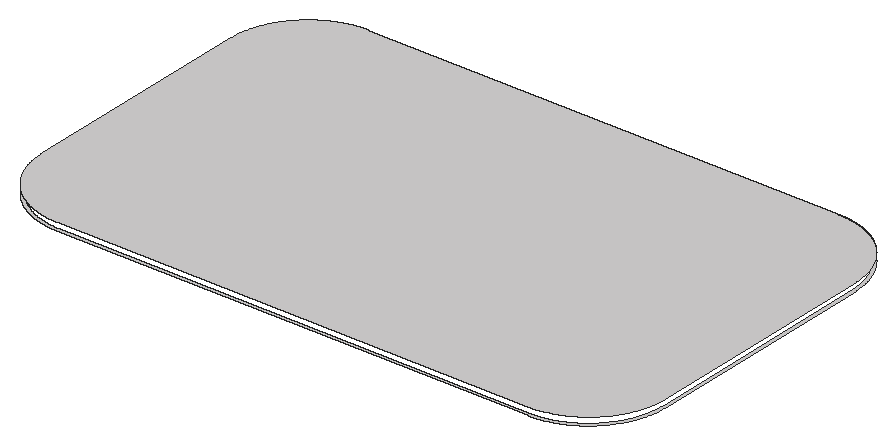
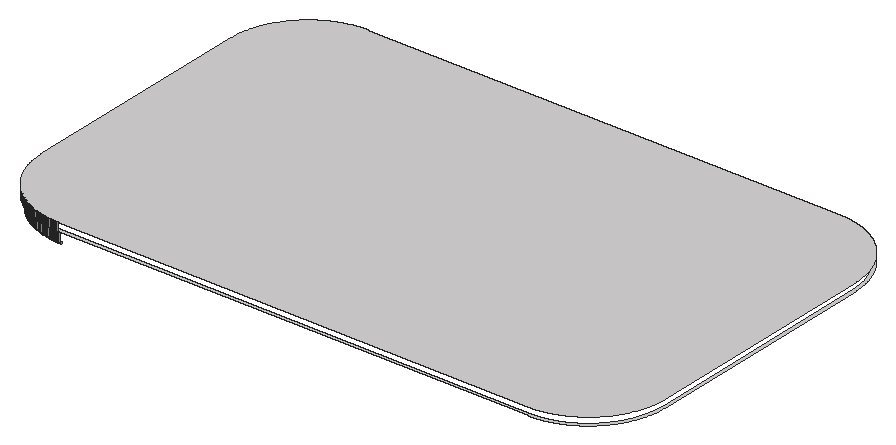
# SketchUp Ruby script. Lengths in inches.
U = 1.inch
M = Sketchup.active_model
def pt(a) = Geom::Point3d.new(a.map { |v| v * U })
def face(e, loops, mat)
  f = e.add_face(loops[0].map { |a| pt(a) })
  loops[1..].each { |l| e.add_face(l.map { |a| pt(a) }).erase! }
  f.material = f.back_material = mat if mat
  f
end
# faces: each face lists its corners as indices into pts; further lists are holes
def faces(e, pts, list, mat = nil) = list.each { |f| face(e, (f[0].is_a?(Array) ? f : [f]).map { |l| l.map { |i| pts[i] } }, mat) }
# xy, xz, yz: faces in a plane at the given z, y or x. An outline is a flat list of corners, or four numbers for a rectangle; further outlines are holes
def ring(l) = l.size == 4 ? [[l[0], l[1]], [l[2], l[1]], [l[2], l[3]], [l[0], l[3]]] : l.each_slice(2).to_a
def flat(e, list, mat, &to3) = list.each { |f| face(e, (f[0].is_a?(Array) ? f : [f]).map { |l| ring(l).map { |u, v| to3.(u, v) } }, mat) }
def xy(e, z, list, mat = nil) = flat(e, list, mat) { |x, y| [x, y, z] }
def xz(e, y, list, mat = nil) = flat(e, list, mat) { |x, z| [x, y, z] }
def yz(e, x, list, mat = nil) = flat(e, list, mat) { |y, z| [x, y, z] }
def lines(e, pts, list) = list.each { |a, b| e.add_line(pt(pts[a]), pt(pts[b])) }
# prism: a flat outline (further loops are holes) pulled along v
def prism(e, loops, v, mat = nil)
  f = face(e, loops, mat); d = Geom::Vector3d.new(v.map { |x| x * U })
  f.pushpull(f.normal.samedirection?(d) ? d.length : -d.length)
end
def box(e, o, s, mat = nil) = prism(e, [[o, [o[0] + s[0], o[1], o[2]], [o[0] + s[0], o[1] + s[1], o[2]], [o[0], o[1] + s[1], o[2]]]], [0, 0, s[2]], mat)
def at(x, y, z, deg = 0) = Geom::Transformation.translation(pt([x, y, z])) * Geom::Transformation.rotation(ORIGIN, Z_AXIS, deg.degrees)
def axes(o, x, y, z) = Geom::Transformation.new([*x, 0, *y, 0, *z, 0, *pt(o).to_a, 1])
def part(name) = M.definitions.add(name)
# library, detail: a bought-in or finely detailed component or shape, given as its bounding box
def library(name, o, s) = part(name).tap { |d| box(d.entities, o, s) }
def detail(e, o, s) = box(e.add_group.entities, o, s)
def put(e, d, t, mat = nil) = e.add_instance(d, t).tap { |i| i.material = mat if mat }
def group(e, t, mat = nil) = e.add_group.tap { |g| g.transformation = t; g.material = mat if mat }.entities
root = M.entities
M.materials.add("[Quartz Light Brown]").color = [215, 212, 212]
xy(root,493,[[[224.48,281.2,223.97,281.21,223.45,281.23,222.93,281.26,222.42,281.29,221.9,281.32,221.39,281.37,220.87,281.42,220.36,281.47,219.84,281.54,219.33,281.61,218.82,281.6875,218.3125,281.77,217.8,281.86,217.29,281.96,216.79,282.0625,216.28,282.17,215.78,282.29,214.28,282.68,213.78,282.83,213.29,282.98,212.79,283.13,211.81,283.47,211.33,283.64,210.84,283.82,210.36,284.01,209.88,284.21,209.41,284.41,208.93,284.62,208.46,284.83,207.99,285.05,207.53,285.27,207.07,285.51,206.61,285.74,206.15,285.99,205.25,286.49,204.8,286.75,203.92,287.29,203.49,287.57,203.05,287.86,202.2,288.44,201.78,288.74,201.37,289.05,200.95,289.36,200.55,289.68,200.14,290,199.74,290.33,199.35,290.66,198.96,291,198.57,291.35,198.1875,291.7,197.81,292.05,197.4375,292.41,197.07,292.77,196.35,293.51,195.99,293.89,195.65,294.27,195.3,294.66,194.96,295.05,194.63,295.44,194.3,295.84,193.98,296.25,193.66,296.65,193.35,297.07,193.04,297.48,192.74,297.9,192.16,298.76,191.87,299.1875,191.59,299.625,191.05,300.5,190.79,300.95,190.29,301.85,190.04,302.31,189.81,302.77,189.57,303.23,189.35,303.7,189.13,304.16,188.91,304.63,188.51,305.59,188.3125,306.0625,188.125,306.55,187.94,307.03,187.77,307.52,187.6,308,187.43,308.49,187.28,308.99,187.125,309.48,186.98,309.98,186.59,311.48,186.47,311.98,186.36,312.49,186.26,312.99,186.16,313.5,186.07,314.01,185.91,315.03,185.84,315.55,185.77,316.06,185.72,316.57,185.67,317.09,185.62,317.6,185.58,318.12,185.55,318.63,185.51,319.67,185.5,320.18,185.5,441.22,185.51,441.73,185.55,442.77,185.58,443.28,185.62,443.8,185.67,444.32,185.77,445.34,185.84,445.86,185.91,446.37,186.07,447.39,186.16,447.9,186.26,448.41,186.36,448.91,186.47,449.42,186.59,449.92,186.98,451.42,187.125,451.92,187.28,452.41,187.43,452.91,187.77,453.89,187.94,454.37,188.125,454.86,188.3125,455.34,188.51,455.82,188.71,456.29,188.91,456.77,189.35,457.71,189.57,458.17,189.81,458.63,190.04,459.09,190.29,459.55,190.79,460.45,191.05,460.9,191.59,461.78,191.87,462.21,192.16,462.65,192.45,463.07,192.74,463.5,193.04,463.92,193.35,464.33,193.66,464.75,193.98,465.16,194.3,465.56,194.63,465.96,194.96,466.35,195.3,466.75,195.65,467.13,195.99,467.51,196.35,467.89,197.07,468.63,197.4375,468.99,197.81,469.35,198.1875,469.71,198.57,470.06,199.35,470.74,199.74,471.07,200.14,471.4,200.55,471.72,200.95,472.04,201.37,472.35,201.78,472.66,202.2,472.96,203.05,473.54,203.49,473.83,203.92,474.11,204.8,474.65,205.25,474.91,206.15,475.41,206.61,475.66,207.07,475.9,207.53,476.13,207.99,476.35,208.93,476.79,209.41,476.99,209.88,477.19,210.36,477.39,210.84,477.58,211.33,477.76,211.81,477.94,212.3,478.1,212.79,478.27,213.29,478.42,213.78,478.57,214.28,478.72,214.78,478.86,215.28,478.99,216.28,479.23,216.79,479.34,217.29,479.44,217.8,479.54,218.3125,479.63,218.82,479.71,219.33,479.79,219.84,479.86,220.36,479.93,220.87,479.98,221.39,480.04,221.9,480.08,222.42,480.12,222.93,480.15,223.45,480.17,223.97,480.1875,224.48,480.2,464.52,480.2,465.03,480.1875,465.55,480.17,466.07,480.15,466.58,480.12,467.1,480.08,467.61,480.04,468.13,479.98,468.64,479.93,469.16,479.86,469.67,479.79,470.18,479.71,470.6875,479.63,471.2,479.54,471.71,479.44,472.21,479.34,472.72,479.23,473.72,478.99,474.22,478.86,474.72,478.72,475.22,478.57,475.71,478.42,476.21,478.27,476.7,478.1,477.19,477.94,477.67,477.76,478.16,477.58,478.64,477.39,479.12,477.19,479.59,476.99,480.07,476.79,481.01,476.35,481.47,476.13,481.93,475.9,482.39,475.66,482.85,475.41,483.75,474.91,484.2,474.65,485.08,474.11,485.51,473.83,485.95,473.54,486.8,472.96,487.22,472.66,487.63,472.35,488.05,472.04,488.45,471.72,488.86,471.4,489.26,471.07,489.65,470.74,490.43,470.06,490.8125,469.71,491.19,469.35,491.5625,468.99,491.93,468.63,492.65,467.89,493.01,467.51,493.35,467.13,493.7,466.75,494.04,466.35,494.37,465.96,494.7,465.56,495.02,465.16,495.34,464.75,495.65,464.33,495.96,463.92,496.26,463.5,496.55,463.07,496.84,462.65,497.13,462.21,497.41,461.78,497.95,460.9,498.21,460.45,498.71,459.55,498.96,459.09,499.19,458.63,499.43,458.17,499.65,457.71,500.09,456.77,500.29,456.29,500.49,455.82,500.6875,455.34,500.875,454.86,501.06,454.37,501.23,453.89,501.57,452.91,501.72,452.41,501.875,451.92,502.02,451.42,502.41,449.92,502.53,449.42,502.64,448.91,502.74,448.41,502.84,447.9,502.93,447.39,503.09,446.37,503.16,445.86,503.23,445.34,503.33,444.32,503.38,443.8,503.42,443.28,503.45,442.77,503.49,441.73,503.5,441.22,503.5,320.18,503.49,319.67,503.45,318.63,503.42,318.12,503.38,317.6,503.33,317.09,503.28,316.57,503.23,316.06,503.16,315.55,503.09,315.03,502.93,314.01,502.84,313.5,502.74,312.99,502.64,312.49,502.53,311.98,502.41,311.48,502.02,309.98,501.875,309.48,501.72,308.99,501.57,308.49,501.4,308,501.23,307.52,501.06,307.03,500.875,306.55,500.6875,306.0625,500.49,305.59,500.09,304.63,499.87,304.16,499.65,303.7,499.43,303.23,499.19,302.77,498.96,302.31,498.71,301.85,498.21,300.95,497.95,300.5,497.41,299.625,497.13,299.1875,496.84,298.76,496.26,297.9,495.96,297.48,495.65,297.07,495.34,296.65,495.02,296.25,494.7,295.84,494.37,295.44,494.04,295.05,493.7,294.66,493.35,294.27,493.01,293.89,492.65,293.51,491.93,292.77,491.5625,292.41,491.19,292.05,490.8125,291.7,490.43,291.35,490.04,291,489.65,290.66,489.26,290.33,488.86,290,488.45,289.68,488.05,289.36,487.63,289.05,487.22,288.74,486.8,288.44,485.95,287.86,485.51,287.57,485.08,287.29,484.2,286.75,483.75,286.49,482.85,285.99,482.39,285.74,481.93,285.51,481.47,285.27,481.01,285.05,480.54,284.83,480.07,284.62,479.59,284.41,479.12,284.21,478.64,284.01,478.16,283.82,477.67,283.64,477.19,283.47,476.21,283.13,475.71,282.98,475.22,282.83,474.72,282.68,473.22,282.29,472.72,282.17,472.21,282.0625,471.71,281.96,471.2,281.86,470.6875,281.77,470.18,281.6875,469.67,281.61,469.16,281.54,468.64,281.47,468.13,281.42,467.61,281.37,467.1,281.32,466.58,281.29,466.07,281.26,465.55,281.23,465.03,281.21,464.52,281.2],[224.5,282.7,464.5,282.7,464.99,282.71,465.99,282.75,466.49,282.78,466.98,282.82,467.48,282.86,467.97,282.91,468.47,282.96,468.96,283.03,469.45,283.09,469.94,283.17,470.44,283.25,470.92,283.34,471.41,283.43,471.9,283.53,472.39,283.64,472.87,283.75,473.35,283.87,473.84,284,474.31,284.13,475.27,284.41,475.74,284.5625,476.21,284.72,476.68,284.88,477.62,285.22,478.08,285.41,478.54,285.59,479.46,285.99,479.91,286.19,480.36,286.4,480.81,286.62,481.25,286.84,481.69,287.07,482.57,287.55,483,287.79,483.43,288.04,483.85,288.3,484.28,288.5625,484.7,288.83,485.11,289.11,485.52,289.38,486.34,289.96,486.74,290.25,487.13,290.55,487.53,290.86,487.91,291.17,488.3,291.49,489.06,292.13,489.43,292.46,489.79,292.8,490.16,293.14,490.52,293.48,491.22,294.18,491.5625,294.54,491.9,294.91,492.24,295.27,492.57,295.65,492.9,296.02,493.22,296.4,494.15,297.57,494.45,297.96,494.74,298.37,495.03,298.77,495.32,299.18,495.6,299.59,495.87,300,496.14,300.42,496.4,300.85,496.66,301.27,496.91,301.7,497.15,302.13,497.4,302.57,497.86,303.45,498.08,303.89,498.3,304.34,498.51,304.79,498.71,305.25,498.91,305.7,499.11,306.16,499.29,306.62,499.48,307.08,499.82,308.02,500.14,308.96,500.29,309.43,500.44,309.91,500.57,310.39,500.71,310.87,500.95,311.83,501.0625,312.31,501.17,312.8,501.27,313.29,501.45,314.27,501.61,315.25,501.67,315.74,501.74,316.23,501.79,316.73,501.84,317.22,501.92,318.22,501.95,318.71,501.99,319.71,502,320.2,502,441.2,501.99,441.7,501.97,442.19,501.95,442.69,501.92,443.1875,501.88,443.68,501.84,444.18,501.79,444.67,501.74,445.17,501.67,445.66,501.61,446.15,501.53,446.65,501.45,447.14,501.27,448.11,501.17,448.6,501.0625,449.09,500.95,449.57,500.83,450.05,500.71,450.54,500.57,451.02,500.44,451.49,500.29,451.97,500.14,452.44,499.98,452.92,499.82,453.39,499.65,453.85,499.48,454.32,499.29,454.78,499.11,455.24,498.71,456.16,498.51,456.61,498.3,457.06,498.08,457.51,497.86,457.95,497.4,458.83,497.15,459.27,496.91,459.7,496.66,460.13,496.4,460.56,496.14,460.98,495.87,461.4,495.6,461.8125,495.32,462.22,494.74,463.04,494.45,463.4375,494.15,463.83,493.84,464.23,493.53,464.62,493.22,465,492.9,465.38,492.57,465.76,492.24,466.13,491.9,466.5,491.5625,466.86,491.22,467.22,490.52,467.92,490.16,468.27,489.79,468.61,489.43,468.94,489.06,469.27,488.68,469.6,488.3,469.92,487.91,470.23,487.53,470.54,487.13,470.85,486.74,471.15,486.34,471.44,485.52,472.02,485.11,472.3,484.7,472.57,484.28,472.84,483.85,473.1,483.43,473.36,482.57,473.86,482.13,474.1,481.25,474.56,480.81,474.78,480.36,475,479.46,475.42,479,475.62,478.08,476,477.62,476.18,476.68,476.52,475.74,476.84,475.27,476.99,474.79,477.14,474.31,477.27,473.84,477.41,473.35,477.53,472.87,477.65,472.39,477.76,471.9,477.87,471.41,477.97,470.92,478.06,470.44,478.15,469.94,478.23,469.45,478.31,468.96,478.375,468.47,478.4375,467.97,478.49,467.48,478.54,466.98,478.58,466.49,478.62,465.99,478.65,465.49,478.67,464.99,478.6875,464.5,478.7,224.5,478.7,224.01,478.6875,223.51,478.67,223.01,478.65,222.51,478.62,222.02,478.58,221.52,478.54,221.03,478.49,220.53,478.4375,220.04,478.375,219.55,478.31,219.06,478.23,218.56,478.15,218.08,478.06,217.59,477.97,217.1,477.87,216.61,477.76,216.13,477.65,215.65,477.53,215.16,477.41,214.69,477.27,214.21,477.14,213.73,476.99,213.26,476.84,212.32,476.52,211.38,476.18,210.92,476,210,475.62,209.54,475.42,208.64,475,208.19,474.78,207.75,474.56,206.87,474.1,206.43,473.86,205.57,473.36,205.15,473.1,204.72,472.84,204.3,472.57,203.89,472.3,203.48,472.02,202.66,471.44,202.26,471.15,201.87,470.85,201.47,470.54,201.09,470.23,200.7,469.92,200.32,469.6,199.94,469.27,199.57,468.94,199.21,468.61,198.84,468.27,198.48,467.92,197.78,467.22,197.4375,466.86,197.1,466.5,196.76,466.13,196.43,465.76,196.1,465.38,195.78,465,195.47,464.62,195.16,464.23,194.85,463.83,194.55,463.4375,194.26,463.04,193.68,462.22,193.4,461.8125,193.13,461.4,192.86,460.98,192.6,460.56,192.34,460.13,192.09,459.7,191.85,459.27,191.6,458.83,191.14,457.95,190.92,457.51,190.7,457.06,190.49,456.61,190.29,456.16,189.89,455.24,189.71,454.78,189.52,454.32,189.35,453.85,189.18,453.39,189.02,452.92,188.86,452.44,188.71,451.97,188.56,451.49,188.43,451.02,188.29,450.54,188.17,450.05,188.05,449.57,187.9375,449.09,187.83,448.6,187.73,448.11,187.55,447.14,187.47,446.65,187.39,446.15,187.33,445.66,187.26,445.17,187.21,444.67,187.16,444.18,187.12,443.68,187.08,443.1875,187.05,442.69,187.03,442.19,187.01,441.7,187,441.2,187,320.2,187.01,319.71,187.05,318.71,187.08,318.22,187.16,317.22,187.21,316.73,187.26,316.23,187.33,315.74,187.39,315.25,187.55,314.27,187.73,313.29,187.83,312.8,187.9375,312.31,188.05,311.83,188.29,310.87,188.43,310.39,188.56,309.91,188.71,309.43,188.86,308.96,189.18,308.02,189.52,307.08,189.71,306.62,189.89,306.16,190.09,305.7,190.29,305.25,190.49,304.79,190.7,304.34,190.92,303.89,191.14,303.45,191.6,302.57,191.85,302.13,192.09,301.7,192.34,301.27,192.6,300.85,192.86,300.42,193.13,300,193.4,299.59,193.68,299.18,193.97,298.77,194.26,298.37,194.55,297.96,194.85,297.57,195.78,296.4,196.1,296.02,196.43,295.65,196.76,295.27,197.1,294.91,197.4375,294.54,197.78,294.18,198.48,293.48,198.84,293.14,199.21,292.8,199.57,292.46,199.94,292.13,200.7,291.49,201.09,291.17,201.47,290.86,201.87,290.55,202.26,290.25,202.66,289.96,203.48,289.38,203.89,289.11,204.3,288.83,204.72,288.5625,205.15,288.3,205.57,288.04,206,287.79,206.43,287.55,207.31,287.07,207.75,286.84,208.19,286.62,208.64,286.4,209.09,286.19,209.54,285.99,210.46,285.59,210.92,285.41,211.38,285.22,212.32,284.88,212.79,284.72,213.26,284.5625,213.73,284.41,214.69,284.13,215.16,284,215.65,283.87,216.13,283.75,216.61,283.64,217.1,283.53,217.59,283.43,218.08,283.34,218.56,283.25,219.06,283.17,219.55,283.09,220.04,283.03,220.53,282.96,221.03,282.91,221.52,282.86,222.02,282.82,222.51,282.78,223.01,282.75,224.01,282.71]]],"[Quartz Light Brown]")
xy(root,497,[[224.48,281.2,464.52,281.2,465.03,281.21,465.55,281.23,466.07,281.26,466.58,281.29,467.1,281.32,467.61,281.37,468.13,281.42,468.64,281.47,469.16,281.54,469.67,281.61,470.18,281.6875,470.6875,281.77,471.2,281.86,471.71,281.96,472.21,282.0625,472.72,282.17,473.22,282.29,474.72,282.68,475.22,282.83,475.71,282.98,476.21,283.13,477.19,283.47,477.67,283.64,478.16,283.82,478.64,284.01,479.12,284.21,479.59,284.41,480.07,284.62,480.54,284.83,481.01,285.05,481.47,285.27,481.93,285.51,482.39,285.74,482.85,285.99,483.75,286.49,484.2,286.75,485.08,287.29,485.51,287.57,485.95,287.86,486.8,288.44,487.22,288.74,487.63,289.05,488.05,289.36,488.45,289.68,488.86,290,489.26,290.33,489.65,290.66,490.04,291,490.43,291.35,490.8125,291.7,491.19,292.05,491.5625,292.41,491.93,292.77,492.65,293.51,493.01,293.89,493.35,294.27,493.7,294.66,494.04,295.05,494.37,295.44,494.7,295.84,495.02,296.25,495.34,296.65,495.65,297.07,495.96,297.48,496.26,297.9,496.84,298.76,497.13,299.1875,497.41,299.625,497.95,300.5,498.21,300.95,498.71,301.85,498.96,302.31,499.19,302.77,499.43,303.23,499.65,303.7,499.87,304.16,500.09,304.63,500.49,305.59,500.6875,306.0625,500.875,306.55,501.06,307.03,501.23,307.52,501.4,308,501.57,308.49,501.72,308.99,501.875,309.48,502.02,309.98,502.41,311.48,502.53,311.98,502.64,312.49,502.74,312.99,502.84,313.5,502.93,314.01,503.09,315.03,503.16,315.55,503.23,316.06,503.28,316.57,503.33,317.09,503.38,317.6,503.42,318.12,503.45,318.63,503.49,319.67,503.5,320.18,503.5,441.22,503.49,441.73,503.45,442.77,503.42,443.28,503.38,443.8,503.33,444.32,503.23,445.34,503.16,445.86,503.09,446.37,502.93,447.39,502.84,447.9,502.74,448.41,502.64,448.91,502.53,449.42,502.41,449.92,502.02,451.42,501.875,451.92,501.72,452.41,501.57,452.91,501.23,453.89,501.06,454.37,500.875,454.86,500.6875,455.34,500.49,455.82,500.29,456.29,500.09,456.77,499.65,457.71,499.43,458.17,499.19,458.63,498.96,459.09,498.71,459.55,498.21,460.45,497.95,460.9,497.41,461.78,497.13,462.21,496.84,462.65,496.55,463.07,496.26,463.5,495.96,463.92,495.65,464.33,495.34,464.75,495.02,465.16,494.7,465.56,494.37,465.96,494.04,466.35,493.7,466.75,493.35,467.13,493.01,467.51,492.65,467.89,491.93,468.63,491.5625,468.99,491.19,469.35,490.8125,469.71,490.43,470.06,489.65,470.74,489.26,471.07,488.86,471.4,488.45,471.72,488.05,472.04,487.63,472.35,487.22,472.66,486.8,472.96,485.95,473.54,485.51,473.83,485.08,474.11,484.2,474.65,483.75,474.91,482.85,475.41,482.39,475.66,481.93,475.9,481.47,476.13,481.01,476.35,480.07,476.79,479.59,476.99,479.12,477.19,478.64,477.39,478.16,477.58,477.67,477.76,477.19,477.94,476.7,478.1,476.21,478.27,475.71,478.42,475.22,478.57,474.72,478.72,474.22,478.86,473.72,478.99,472.72,479.23,472.21,479.34,471.71,479.44,471.2,479.54,470.6875,479.63,470.18,479.71,469.67,479.79,469.16,479.86,468.64,479.93,468.13,479.98,467.61,480.04,467.1,480.08,466.58,480.12,466.07,480.15,465.55,480.17,465.03,480.1875,464.52,480.2,224.48,480.2,223.97,480.1875,223.45,480.17,222.93,480.15,222.42,480.12,221.9,480.08,221.39,480.04,220.87,479.98,220.36,479.93,219.84,479.86,219.33,479.79,218.82,479.71,218.3125,479.63,217.8,479.54,217.29,479.44,216.79,479.34,216.28,479.23,215.28,478.99,214.78,478.86,214.28,478.72,213.78,478.57,213.29,478.42,212.79,478.27,212.3,478.1,211.81,477.94,211.33,477.76,210.84,477.58,210.36,477.39,209.88,477.19,209.41,476.99,208.93,476.79,207.99,476.35,207.53,476.13,207.07,475.9,206.61,475.66,206.15,475.41,205.25,474.91,204.8,474.65,203.92,474.11,203.49,473.83,203.05,473.54,202.2,472.96,201.78,472.66,201.37,472.35,200.95,472.04,200.55,471.72,200.14,471.4,199.74,471.07,199.35,470.74,198.57,470.06,198.1875,469.71,197.81,469.35,197.4375,468.99,197.07,468.63,196.35,467.89,195.99,467.51,195.65,467.13,195.3,466.75,194.96,466.35,194.63,465.96,194.3,465.56,193.98,465.16,193.66,464.75,193.35,464.33,193.04,463.92,192.74,463.5,192.45,463.07,192.16,462.65,191.87,462.21,191.59,461.78,191.05,460.9,190.79,460.45,190.29,459.55,190.04,459.09,189.81,458.63,189.57,458.17,189.35,457.71,188.91,456.77,188.71,456.29,188.51,455.82,188.3125,455.34,188.125,454.86,187.94,454.37,187.77,453.89,187.43,452.91,187.28,452.41,187.125,451.92,186.98,451.42,186.59,449.92,186.47,449.42,186.36,448.91,186.26,448.41,186.16,447.9,186.07,447.39,185.91,446.37,185.84,445.86,185.77,445.34,185.67,444.32,185.62,443.8,185.58,443.28,185.55,442.77,185.51,441.73,185.5,441.22,185.5,320.18,185.51,319.67,185.55,318.63,185.58,318.12,185.62,317.6,185.67,317.09,185.72,316.57,185.77,316.06,185.84,315.55,185.91,315.03,186.07,314.01,186.16,313.5,186.26,312.99,186.36,312.49,186.47,311.98,186.59,311.48,186.98,309.98,187.125,309.48,187.28,308.99,187.43,308.49,187.6,308,187.77,307.52,187.94,307.03,188.125,306.55,188.3125,306.0625,188.51,305.59,188.91,304.63,189.13,304.16,189.35,303.7,189.57,303.23,189.81,302.77,190.04,302.31,190.29,301.85,190.79,300.95,191.05,300.5,191.59,299.625,191.87,299.1875,192.16,298.76,192.74,297.9,193.04,297.48,193.35,297.07,193.66,296.65,193.98,296.25,194.3,295.84,194.63,295.44,194.96,295.05,195.3,294.66,195.65,294.27,195.99,293.89,196.35,293.51,197.07,292.77,197.4375,292.41,197.81,292.05,198.1875,291.7,198.57,291.35,198.96,291,199.35,290.66,199.74,290.33,200.14,290,200.55,289.68,200.95,289.36,201.37,289.05,201.78,288.74,202.2,288.44,203.05,287.86,203.49,287.57,203.92,287.29,204.8,286.75,205.25,286.49,206.15,285.99,206.61,285.74,207.07,285.51,207.53,285.27,207.99,285.05,208.46,284.83,208.93,284.62,209.41,284.41,209.88,284.21,210.36,284.01,210.84,283.82,211.33,283.64,211.81,283.47,212.79,283.13,213.29,282.98,213.78,282.83,214.28,282.68,215.78,282.29,216.28,282.17,216.79,282.0625,217.29,281.96,217.8,281.86,218.3125,281.77,218.82,281.6875,219.33,281.61,219.84,281.54,220.36,281.47,220.87,281.42,221.39,281.37,221.9,281.32,222.42,281.29,222.93,281.26,223.45,281.23,223.97,281.21]],"[Quartz Light Brown]")
xz(root,477.7,[[464,486,464.48,487]],"[Quartz Light Brown]")
xz(root,478.7,[[464,487,464.5,493]],"[Quartz Light Brown]")
xz(root,480.2,[[464,493,464.52,497]],"[Quartz Light Brown]")
p = [[490.84,466.17,486],[490.5,466.52,486],[490.5,466.52,487],[490.84,466.17,487],[490.16,466.86,486],[490.16,466.86,487],
  [489.82,467.2,486],[489.82,467.2,487],[489.47,467.54,486],[489.47,467.54,487],[489.12,467.87,486],[489.12,467.87,487],
  [488.76,468.2,486],[488.76,468.2,487],[488.4,468.52,486],[488.4,468.52,487],[488.03,468.84,486],[488.03,468.84,487],
  [487.66,469.15,486],[487.66,469.15,487],[487.28,469.46,486],[487.28,469.46,487],[486.91,469.76,486],[486.91,469.76,487],
  [486.52,470.06,486],[486.52,470.06,487],[486.14,470.35,486],[486.14,470.35,487],[485.75,470.63,486],[485.75,470.63,487],
  [485.35,470.92,486],[485.35,470.92,487],[484.96,471.19,486],[484.96,471.19,487],[484.56,471.47,486],[484.56,471.47,487],
  [484.15,471.73,486],[484.15,471.73,487],[483.74,471.99,486],[483.74,471.99,487],[483.33,472.25,486],[483.33,472.25,487],
  [482.92,472.5,486],[482.92,472.5,487],[482.5,472.74,486],[482.5,472.74,487],[482.08,472.98,486],[482.08,472.98,487],
  [481.65,473.22,486],[481.65,473.22,487],[481.23,473.45,486],[481.23,473.45,487],[480.8,473.67,486],[480.8,473.67,487],
  [480.36,473.89,486],[480.36,473.89,487],[479.93,474.1,486],[479.93,474.1,487],[479.49,474.3,486],[479.49,474.3,487],
  [479.05,474.5,486],[479.05,474.5,487],[478.61,474.7,486],[478.61,474.7,487],[478.16,474.88,486],[478.16,474.88,487],
  [477.71,475.07,486],[477.71,475.07,487],[477.26,475.24,486],[477.26,475.24,487],[476.81,475.41,486],[476.81,475.41,487],
  [476.35,475.58,486],[476.35,475.58,487],[475.89,475.74,486],[475.89,475.74,487],[475.43,475.89,486],[475.43,475.89,487],
  [474.97,476.04,486],[474.97,476.04,487],[474.51,476.18,486],[474.51,476.18,487],[474.04,476.3125,486],[474.04,476.3125,487],
  [473.58,476.44,486],[473.58,476.44,487],[473.11,476.5625,486],[473.11,476.5625,487],[472.64,476.68,486],[472.64,476.68,487],
  [472.17,476.79,486],[472.17,476.79,487],[471.69,476.89,486],[471.69,476.89,487],[471.22,476.99,486],[471.22,476.99,487],
  [470.74,477.08,486],[470.74,477.08,487],[470.27,477.17,486],[470.27,477.17,487],[469.79,477.25,486],[469.31,477.32,486],
  [469.31,477.32,487],[469.79,477.25,487],[468.83,477.38,486],[468.83,477.38,487],[468.35,477.44,486],[467.87,477.5,486],
  [467.87,477.5,487],[468.35,477.44,487],[467.39,477.55,486],[466.9,477.59,486],[466.9,477.59,487],[467.39,477.55,487],
  [466.42,477.62,486],[465.9375,477.65,486],[465.9375,477.65,487],[466.42,477.62,487],[464.97,477.6875,486],[464.48,477.7,486],
  [464.48,477.7,487],[464.97,477.6875,487],[465.45,477.67,486],[465.45,477.67,487],[490.52,467.92,487],[490.52,467.92,493],
  [490.87,467.57,493],[490.87,467.57,487],[490.16,468.27,487],[490.16,468.27,493],[489.79,468.61,487],[489.79,468.61,493],
  [489.43,468.94,487],[489.43,468.94,493],[489.06,469.27,487],[489.06,469.27,493],[488.68,469.6,487],[488.68,469.6,493],
  [488.3,469.92,487],[488.3,469.92,493],[487.91,470.23,487],[487.91,470.23,493],[487.53,470.54,487],[487.53,470.54,493],
  [487.13,470.85,487],[487.13,470.85,493],[486.74,471.15,487],[486.74,471.15,493],[486.34,471.44,487],[486.34,471.44,493],
  [485.93,471.73,487],[485.93,471.73,493],[485.52,472.02,487],[485.52,472.02,493],[485.11,472.3,487],[485.11,472.3,493],
  [484.7,472.57,487],[484.7,472.57,493],[484.28,472.84,487],[484.28,472.84,493],[483.85,473.1,487],[483.85,473.1,493],
  [483.43,473.36,487],[483.43,473.36,493],[483,473.61,487],[483,473.61,493],[482.57,473.86,487],[482.57,473.86,493],
  [482.13,474.1,487],[482.13,474.1,493],[481.69,474.33,487],[481.69,474.33,493],[481.25,474.56,487],[481.25,474.56,493],
  [480.81,474.78,487],[480.81,474.78,493],[480.36,475,487],[480.36,475,493],[479.91,475.21,487],[479.91,475.21,493],
  [479.46,475.42,487],[479.46,475.42,493],[479,475.62,487],[479,475.62,493],[478.54,475.81,487],[478.54,475.81,493],
  [478.08,476,487],[478.08,476,493],[477.62,476.18,487],[477.62,476.18,493],[477.15,476.35,487],[477.15,476.35,493],
  [476.68,476.52,487],[476.68,476.52,493],[476.21,476.68,487],[476.21,476.68,493],[475.74,476.84,487],[475.74,476.84,493],
  [475.27,476.99,487],[475.27,476.99,493],[474.79,477.14,487],[474.79,477.14,493],[474.31,477.27,487],[474.31,477.27,493],
  [473.84,477.41,487],[473.84,477.41,493],[473.35,477.53,487],[473.35,477.53,493],[472.87,477.65,487],[472.87,477.65,493],
  [472.39,477.76,487],[472.39,477.76,493],[471.9,477.87,487],[471.9,477.87,493],[471.41,477.97,487],[471.41,477.97,493],
  [470.92,478.06,487],[470.92,478.06,493],[470.44,478.15,487],[470.44,478.15,493],[469.45,478.31,487],[469.45,478.31,493],
  [469.94,478.23,493],[469.94,478.23,487],[468.96,478.375,487],[468.96,478.375,493],[467.97,478.49,487],[467.97,478.49,493],
  [468.47,478.4375,493],[468.47,478.4375,487],[466.98,478.58,487],[466.98,478.58,493],[467.48,478.54,493],[467.48,478.54,487],
  [465.49,478.67,487],[465.49,478.67,493],[465.99,478.65,493],[465.99,478.65,487],[466.49,478.62,493],[466.49,478.62,487],
  [464.5,478.7,487],[464.5,478.7,493],[464.99,478.6875,493],[464.99,478.6875,487],[491.19,469.35,493],[490.8125,469.71,493],
  [490.8125,469.71,497],[491.19,469.35,497],[490.43,470.06,493],[490.43,470.06,497],[490.04,470.4,493],[490.04,470.4,497],
  [489.65,470.74,493],[489.65,470.74,497],[489.26,471.07,493],[489.26,471.07,497],[488.86,471.4,493],[488.86,471.4,497],
  [488.45,471.72,493],[488.45,471.72,497],[488.05,472.04,493],[488.05,472.04,497],[487.63,472.35,493],[487.63,472.35,497],
  [487.22,472.66,493],[487.22,472.66,497],[486.8,472.96,493],[486.8,472.96,497],[486.375,473.25,493],[486.375,473.25,497],
  [485.95,473.54,493],[485.95,473.54,497],[485.51,473.83,493],[485.51,473.83,497],[485.08,474.11,493],[485.08,474.11,497],
  [484.64,474.38,493],[484.64,474.38,497],[484.2,474.65,493],[484.2,474.65,497],[483.75,474.91,493],[483.75,474.91,497],
  [483.3,475.16,493],[483.3,475.16,497],[482.85,475.41,493],[482.85,475.41,497],[482.39,475.66,493],[482.39,475.66,497],
  [481.93,475.9,493],[481.93,475.9,497],[481.47,476.13,493],[481.47,476.13,497],[481.01,476.35,493],[481.01,476.35,497],
  [480.54,476.57,493],[480.54,476.57,497],[480.07,476.79,493],[480.07,476.79,497],[479.59,476.99,493],[479.59,476.99,497],
  [479.12,477.19,493],[479.12,477.19,497],[478.64,477.39,493],[478.64,477.39,497],[478.16,477.58,493],[478.16,477.58,497],
  [477.67,477.76,493],[477.67,477.76,497],[477.19,477.94,493],[477.19,477.94,497],[476.7,478.1,493],[476.7,478.1,497],
  [476.21,478.27,493],[476.21,478.27,497],[475.71,478.42,493],[475.71,478.42,497],[475.22,478.57,493],[475.22,478.57,497],
  [474.72,478.72,493],[474.72,478.72,497],[474.22,478.86,493],[474.22,478.86,497],[473.72,478.99,493],[473.72,478.99,497],
  [473.22,479.11,493],[473.22,479.11,497],[472.72,479.23,493],[472.72,479.23,497],[472.21,479.34,493],[472.21,479.34,497],
  [471.71,479.44,493],[471.71,479.44,497],[471.2,479.54,493],[471.2,479.54,497],[470.6875,479.63,493],[470.6875,479.63,497],
  [470.18,479.71,493],[470.18,479.71,497],[469.67,479.79,493],[469.67,479.79,497],[469.16,479.86,493],[469.16,479.86,497],
  [468.64,479.93,493],[468.13,479.98,493],[468.13,479.98,497],[468.64,479.93,497],[467.61,480.04,493],[467.1,480.08,493],
  [467.1,480.08,497],[467.61,480.04,497],[466.07,480.15,493],[465.55,480.17,493],[465.55,480.17,497],[466.07,480.15,497],
  [466.58,480.12,493],[466.58,480.12,497],[465.03,480.1875,493],[464.52,480.2,493],[464.52,480.2,497],[465.03,480.1875,497],
  [464,478.7,493],[464,478.7,495]]
faces(root,p,[[0,1,2,3],[1,4,5,2],[4,6,7,5],[6,8,9,7],[8,10,11,9],[10,12,13,11],[12,14,15,13],[14,16,17,15],
  [16,18,19,17],[18,20,21,19],[20,22,23,21],[22,24,25,23],[24,26,27,25],[26,28,29,27],[28,30,31,29],[30,32,33,31],
  [32,34,35,33],[34,36,37,35],[36,38,39,37],[38,40,41,39],[40,42,43,41],[42,44,45,43],[44,46,47,45],[46,48,49,47],
  [48,50,51,49],[50,52,53,51],[52,54,55,53],[54,56,57,55],[56,58,59,57],[58,60,61,59],[60,62,63,61],[62,64,65,63],
  [64,66,67,65],[66,68,69,67],[68,70,71,69],[70,72,73,71],[72,74,75,73],[74,76,77,75],[76,78,79,77],[78,80,81,79],
  [80,82,83,81],[82,84,85,83],[84,86,87,85],[86,88,89,87],[88,90,91,89],[90,92,93,91],[92,94,95,93],[94,96,97,95],
  [96,98,99,97],[100,101,102,103],[98,100,103,99],[101,104,105,102],[106,107,108,109],[104,106,109,105],[110,111,112,113],[107,110,113,108],
  [114,115,116,117],[111,114,117,112],[118,119,120,121],[122,118,121,123],[115,122,123,116],[124,125,126,127],[128,129,125,124],[130,131,129,128],
  [132,133,131,130],[134,135,133,132],[136,137,135,134],[138,139,137,136],[140,141,139,138],[142,143,141,140],[144,145,143,142],[146,147,145,144],
  [148,149,147,146],[150,151,149,148],[152,153,151,150],[154,155,153,152],[156,157,155,154],[158,159,157,156],[160,161,159,158],[162,163,161,160],
  [164,165,163,162],[166,167,165,164],[168,169,167,166],[170,171,169,168],[172,173,171,170],[174,175,173,172],[176,177,175,174],[178,179,177,176],
  [180,181,179,178],[182,183,181,180],[184,185,183,182],[186,187,185,184],[188,189,187,186],[190,191,189,188],[192,193,191,190],[194,195,193,192],
  [196,197,195,194],[198,199,197,196],[200,201,199,198],[202,203,201,200],[204,205,203,202],[206,207,205,204],[208,209,207,206],[210,211,209,208],
  [212,213,211,210],[214,215,213,212],[216,217,215,214],[218,219,217,216],[220,221,222,223],[223,222,219,218],[224,225,221,220],[226,227,228,229],
  [229,228,225,224],[230,231,232,233],[233,232,227,226],[234,235,236,237],[237,236,238,239],[239,238,231,230],[240,241,242,243],[243,242,235,234],
  [244,245,246,247],[245,248,249,246],[248,250,251,249],[250,252,253,251],[252,254,255,253],[254,256,257,255],[256,258,259,257],[258,260,261,259],
  [260,262,263,261],[262,264,265,263],[264,266,267,265],[266,268,269,267],[268,270,271,269],[270,272,273,271],[272,274,275,273],[274,276,277,275],
  [276,278,279,277],[278,280,281,279],[280,282,283,281],[282,284,285,283],[284,286,287,285],[286,288,289,287],[288,290,291,289],[290,292,293,291],
  [292,294,295,293],[294,296,297,295],[296,298,299,297],[298,300,301,299],[300,302,303,301],[302,304,305,303],[304,306,307,305],[306,308,309,307],
  [308,310,311,309],[310,312,313,311],[312,314,315,313],[314,316,317,315],[316,318,319,317],[318,320,321,319],[320,322,323,321],[322,324,325,323],
  [324,326,327,325],[326,328,329,327],[328,330,331,329],[330,332,333,331],[332,334,335,333],[334,336,337,335],[336,338,339,337],[338,340,341,339],
  [342,343,344,345],[340,342,345,341],[346,347,348,349],[343,346,349,344],[350,351,352,353],[354,350,353,355],[347,354,355,348],[356,357,358,359],
  [351,356,359,352]],"[Quartz Light Brown]")
lines(root,p,[[360,361]])
